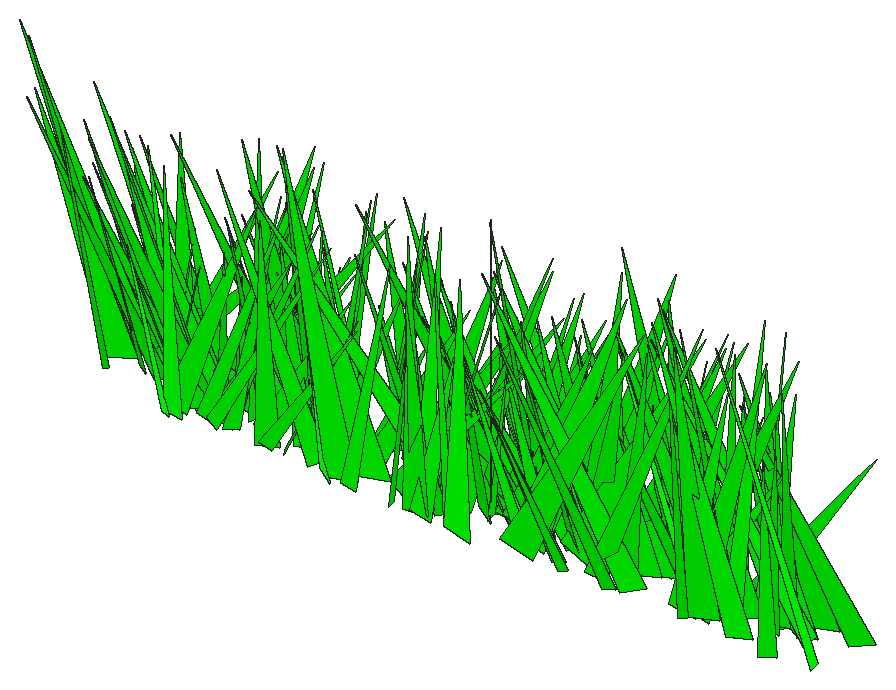
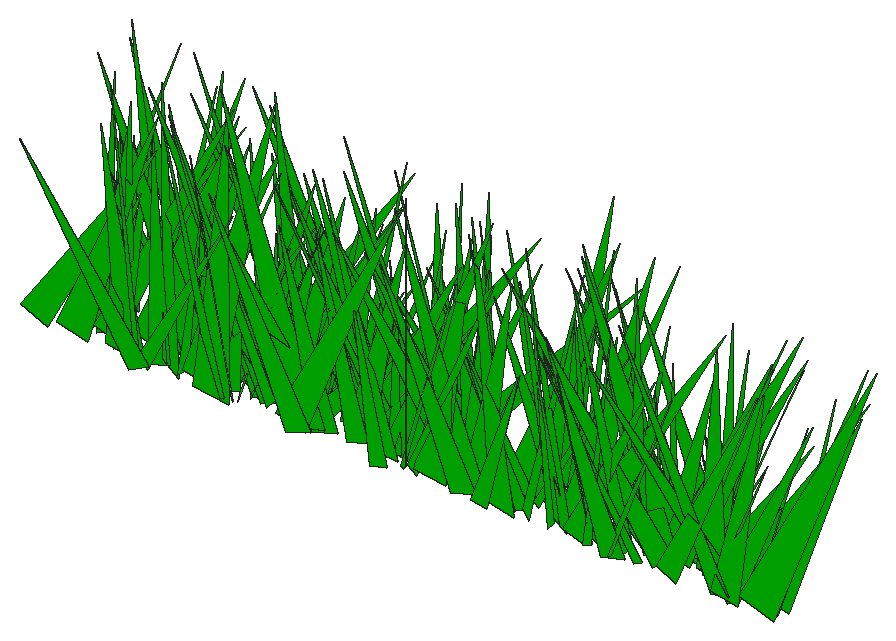
# SketchUp Ruby script. Lengths in inches.
U = 1.inch
M = Sketchup.active_model
def pt(a) = Geom::Point3d.new(a.map { |v| v * U })
def face(e, loops, mat)
  f = e.add_face(loops[0].map { |a| pt(a) })
  loops[1..].each { |l| e.add_face(l.map { |a| pt(a) }).erase! }
  f.material = f.back_material = mat if mat
  f
end
# faces: each face lists its corners as indices into pts; further lists are holes
def faces(e, pts, list, mat = nil) = list.each { |f| face(e, (f[0].is_a?(Array) ? f : [f]).map { |l| l.map { |i| pts[i] } }, mat) }
# xy, xz, yz: faces in a plane at the given z, y or x. An outline is a flat list of corners, or four numbers for a rectangle; further outlines are holes
def ring(l) = l.size == 4 ? [[l[0], l[1]], [l[2], l[1]], [l[2], l[3]], [l[0], l[3]]] : l.each_slice(2).to_a
def flat(e, list, mat, &to3) = list.each { |f| face(e, (f[0].is_a?(Array) ? f : [f]).map { |l| ring(l).map { |u, v| to3.(u, v) } }, mat) }
def xy(e, z, list, mat = nil) = flat(e, list, mat) { |x, y| [x, y, z] }
def xz(e, y, list, mat = nil) = flat(e, list, mat) { |x, z| [x, y, z] }
def yz(e, x, list, mat = nil) = flat(e, list, mat) { |y, z| [x, y, z] }
def lines(e, pts, list) = list.each { |a, b| e.add_line(pt(pts[a]), pt(pts[b])) }
# prism: a flat outline (further loops are holes) pulled along v
def prism(e, loops, v, mat = nil)
  f = face(e, loops, mat); d = Geom::Vector3d.new(v.map { |x| x * U })
  f.pushpull(f.normal.samedirection?(d) ? d.length : -d.length)
end
def box(e, o, s, mat = nil) = prism(e, [[o, [o[0] + s[0], o[1], o[2]], [o[0] + s[0], o[1] + s[1], o[2]], [o[0], o[1] + s[1], o[2]]]], [0, 0, s[2]], mat)
def at(x, y, z, deg = 0) = Geom::Transformation.translation(pt([x, y, z])) * Geom::Transformation.rotation(ORIGIN, Z_AXIS, deg.degrees)
def axes(o, x, y, z) = Geom::Transformation.new([*x, 0, *y, 0, *z, 0, *pt(o).to_a, 1])
def part(name) = M.definitions.add(name)
# library, detail: a bought-in or finely detailed component or shape, given as its bounding box
def library(name, o, s) = part(name).tap { |d| box(d.entities, o, s) }
def detail(e, o, s) = box(e.add_group.entities, o, s)
def put(e, d, t, mat = nil) = e.add_instance(d, t).tap { |i| i.material = mat if mat }
def group(e, t, mat = nil) = e.add_group.tap { |g| g.transformation = t; g.material = mat if mat }.entities
root = M.entities
M.materials.add("[0065_Lime]").color = [0, 255, 0]
c1 = part("fur_instance\#9")
p = [[0.8125,0,1.79],[0.67,-0.02,1.48],[0,-0.11,0],[0,0.11,0]]
faces(c1.entities,p,[[0,1,2,3]])
put(root,c1,axes([8.35,30.09,1.48],[-0.97184,-1.14595,3.29784],[8.52533,0.08708,2.67617],[-3.20375,0.57933,6.12105]),"[0065_Lime]")
put(root,c1,axes([8.03,29.625,1.48],[-7.32027,-0.64299,1.47519],[4.91342,-0.98176,1.79282],[0.29309,0.39896,6.7893]),"[0065_Lime]")
put(root,c1,axes([8.07,29.26,1.48],[-0.99814,1.05656,0.62338],[-7.15463,-0.09708,-2.06636],[-2.43606,-0.1478,5.81341]),"[0065_Lime]")
put(root,c1,axes([8.03,28.19,1.48],[-6.15676,-0.26004,1.50467],[2.26605,-0.86217,1.14185],[1.30829,0.26959,5.10315]),"[0065_Lime]")
put(root,c1,axes([10.48,28.9,1.48],[-6.27578,-0.65891,0.1631],[4.53982,-0.84028,1.82705],[-1.191,0.26908,6.10485]),"[0065_Lime]")
put(root,c1,axes([9.92,29.98,1.48],[-4.83605,-0.60584,1.73783],[4.78748,-0.56307,2.23707],[-0.48321,0.48463,4.77167]),"[0065_Lime]")
put(root,c1,axes([9.3,29.0625,1.48],[-5.32084,-0.29493,0.50758],[1.94317,-0.7422,-0.97326],[1.0093,-0.12587,4.54965]),"[0065_Lime]")
put(root,c1,axes([11.53,29.21,1.48],[-2.23326,-0.7401,0.77563],[4.95786,-0.2313,2.04934],[-2.01734,0.25086,4.17786]),"[0065_Lime]")
put(root,c1,axes([9.94,30.27,1.48],[1.48633,-0.93311,0.42277],[6.47605,0.21995,1.20288],[-1.55812,0.02405,5.40287]),"[0065_Lime]")
put(root,c1,axes([10.84,29.81,1.48],[-4.63654,0.19619,0.01665],[-1.34515,-0.63022,1.00372],[0.37476,0.16523,3.80867]),"[0065_Lime]")
put(root,c1,axes([12.09,28.28,1.48],[-7.31753,-0.35366,0.04909],[2.26762,-0.93721,-2.60519],[1.09369,-0.42308,5.72998]),"[0065_Lime]")
put(root,c1,axes([12.22,28.89,1.48],[-4.77681,-0.10309,0.28654],[0.81372,-0.59945,1.74818],[-0.01527,0.30602,3.52098]),"[0065_Lime]")
put(root,c1,axes([13.86,28.35,1.48],[-3.58464,1.16781,0.62225],[-8.02183,-0.44983,-2.28713],[-2.30306,-0.25086,6.99782]),"[0065_Lime]")
put(root,c1,axes([13.09,30.21,1.48],[-4.46996,-0.70372,1.31461],[5.21048,-0.55011,1.85446],[-0.73726,0.37878,5.13569]),"[0065_Lime]")
put(root,c1,axes([13.71,27.94,1.48],[-3.83914,-0.9369,0.49014],[6.48063,-0.49562,1.84029],[-1.67926,0.22925,5.98153]),"[0065_Lime]")
put(root,c1,axes([11.9,28.12,1.48],[-6.67185,0.3202,1.33269],[-2.00766,-0.9594,1.074],[1.96115,0.10716,5.6333]),"[0065_Lime]")
put(root,c1,axes([13.56,28.91,1.48],[-4.31946,0.82738,1.28636],[-6.02935,-0.53932,-1.77163],[-0.90401,-0.35625,5.66963]),"[0065_Lime]")
put(root,c1,axes([13.8,27.97,1.48],[-7.33696,-0.45983,1.01519],[3.49568,-0.98653,1.74213],[0.2157,0.347,6.29818]),"[0065_Lime]")
put(root,c1,axes([13.24,27.84,1.48],[-2.73427,0.90347,0.68486],[-6.37937,-0.35176,-1.30181],[-1.1627,-0.19463,5.53206]),"[0065_Lime]")
put(root,c1,axes([11.55,29.11,1.48],[2.14592,1.02268,0.75275],[-7.19215,0.31999,-1.00192],[-1.44846,-0.07376,6.09009]),"[0065_Lime]")
put(root,c1,axes([12.44,26.65,1.48],[-4.62827,0.19644,0.38265],[-1.25208,-0.63831,0.96033],[0.77968,0.14103,3.81362]),"[0065_Lime]")
put(root,c1,axes([11.1,28.67,1.48],[4.72564,0.21525,1.01076],[-1.0953,0.66336,-1.34548],[-1.64038,0.17715,3.81021]),"[0065_Lime]")
put(root,c1,axes([11.51,28.17,1.48],[4.07647,0.10586,0.77597],[-0.4582,0.56832,-1.00527],[-1.12588,0.15198,3.21866]),"[0065_Lime]")
put(root,c1,axes([12.72,26.81,1.48],[-6.19282,0.53477,1.31474],[-3.46206,-0.89428,1.39905],[2.26049,0.09541,5.74456]),"[0065_Lime]")
put(root,c1,axes([13.95,28.97,1.48],[1.44044,0.80035,1.96536],[-5.80563,0.29535,-1.21496],[-2.13868,-0.2627,4.62182]),"[0065_Lime]")
put(root,c1,axes([10.24,30.18,1.48],[5.66866,0.67536,0.71281],[-4.86771,0.76473,1.33372],[0.41577,-0.25463,5.89625]),"[0065_Lime]")
put(root,c1,axes([9.47,30,1.48],[5.43307,-0.59886,0.16116],[3.76874,0.65253,-2.81213],[1.99968,0.39726,4.86207]),"[0065_Lime]")
put(root,c1,axes([12.39,27.36,1.48],[3.44675,0.87455,0.94011],[-6.28399,0.45041,1.20327],[0.76337,-0.24099,5.66052]),"[0065_Lime]")
put(root,c1,axes([18.15,29.45,1.48],[-4.90993,-0.95425,0.12481],[6.5341,-0.65623,1.94955],[-1.85645,0.2141,6.53168]),"[0065_Lime]")
put(root,c1,axes([16.02,30.52,1.48],[-5.37657,-0.32663,0.09773],[2.19306,-0.72512,-1.38198],[0.77991,-0.21277,4.55978]),"[0065_Lime]")
put(root,c1,axes([14.16,28.37,1.48],[-4.55313,-0.58157,0.58505],[3.37137,-0.59481,-2.45291],[2.50612,-0.25644,4.36271]),"[0065_Lime]")
put(root,c1,axes([15.73,28.78,1.48],[6.82093,0.89005,0.74167],[-5.21382,0.88151,-3.7221],[-3.71052,0.3975,6.59349]),"[0065_Lime]")
put(root,c1,axes([15.48,27.5,1.48],[-4.21522,-0.04002,1.81893],[1.21862,-0.60101,1.42536],[1.89645,0.29724,3.127]),"[0065_Lime]")
put(root,c1,axes([13.24,28.53,1.48],[2.38102,-0.7524,0.33874],[5.15504,0.30222,-1.48046],[1.50641,0.155,4.53086]),"[0065_Lime]")
put(root,c1,axes([16.4375,28.5,1.48],[-6.08492,-0.64352,0.02362],[4.08332,-0.76542,-2.77695],[2.07369,-0.3811,5.53742]),"[0065_Lime]")
put(root,c1,axes([14.15,28.06,1.48],[2.05348,0.47895,0.93099],[-3.46149,0.21325,1.37543],[0.97245,-0.25229,2.92999]),"[0065_Lime]")
put(root,c1,axes([14.45,28.41,1.48],[-1.7297,0.78278,1.62237],[-5.40952,-0.32752,1.47931],[2.39753,-0.17423,4.5082]),"[0065_Lime]")
put(root,c1,axes([13.8125,28.89,1.48],[-2.12175,1.24777,1.08071],[-8.35474,-0.34463,2.48067],[3.28848,-0.07051,6.99969]),"[0065_Lime]")
put(root,c1,axes([13.96,27.4,1.48],[6.93903,-0.34959,1.35721],[2.87332,0.94403,-1.57158],[-0.84716,0.33839,5.7865]),"[0065_Lime]")
put(root,c1,axes([18.26,30.02,1.48],[-3.06513,-0.7045,0.61286],[4.978,-0.39475,1.26721],[-0.96112,0.20222,4.60887]),"[0065_Lime]")
put(root,c1,axes([15.41,27.34,1.48],[6.18285,0.7193,0.29128],[-4.82277,0.84146,-1.89736],[-1.75296,0.22202,6.24744]),"[0065_Lime]")
put(root,c1,axes([14.22,29.12,1.48],[1.43022,-1.18718,1.37587],[8.39868,0.13828,-1.77822],[1.92406,0.27886,6.73932]),"[0065_Lime]")
put(root,c1,axes([15.625,29.73,1.48],[7.6016,-0.16949,2.30745],[2.19241,1.04292,-2.21185],[-2.16687,0.46063,5.85686]),"[0065_Lime]")
put(root,c1,axes([17.32,30.27,1.48],[-5.76029,-0.40293,1.31263],[2.52516,-0.83445,-1.25126],[2.10948,-0.10138,5.08217]),"[0065_Lime]")
put(root,c1,axes([18.84,28.96,1.48],[-0.27338,-1.28528,0.61899],[8.99873,-0.01647,1.48349],[-1.80699,0.11242,7.29409]),"[0065_Lime]")
put(root,c1,axes([14.67,30.15,1.48],[5.23159,0.37079,0.12512],[-2.54466,0.69356,1.52598],[0.71503,-0.24467,4.51521]),"[0065_Lime]")
put(root,c1,axes([15,27.53,1.48],[7.1417,-0.28239,0.71473],[2.13405,0.99175,-0.97858],[-0.50648,0.19687,5.95489]),"[0065_Lime]")
put(root,c1,axes([17.51,27.16,1.48],[4.30859,-0.79145,1.16125],[5.47964,0.63653,1.0851],[-1.93272,0.04031,5.66524]),"[0065_Lime]")
put(root,c1,axes([20.11,27.35,1.48],[-7.23972,0.53248,2.02561],[-4.50893,-0.91517,-2.60122],[0.48002,-0.56553,6.11665]),"[0065_Lime]")
put(root,c1,axes([14.48,27.2,1.48],[6.67903,0.45508,0.10268],[-3.19482,0.9176,1.22384],[0.54532,-0.19784,5.91246]),"[0065_Lime]")
put(root,c1,axes([15.73,30.5,1.48],[1.529,-0.82776,0.08876],[5.69209,0.20344,-1.3002],[1.52098,0.07076,4.77662]),"[0065_Lime]")
put(root,c1,axes([18.83,28.04,1.48],[1.6355,0.7903,1.11266],[-5.53641,0.27186,-1.08601],[-1.68842,-0.12591,4.63887]),"[0065_Lime]")
put(root,c1,axes([13.81,29.5,1.48],[6.8052,-0.67836,0.68488],[4.63338,0.82476,-3.0874],[1.59572,0.49818,6.04392]),"[0065_Lime]")
put(root,c1,axes([17.36,29.91,1.48],[4.84983,0.15697,0.90715],[-0.78141,0.6787,-1.17119],[-1.3715,0.16838,3.87509]),"[0065_Lime]")
put(root,c1,axes([19.34,28.12,1.48],[-7.66578,-0.29747,2.32532],[2.66286,-1.11263,1.03878],[2.35858,0.28935,6.38489]),"[0065_Lime]")
put(root,c1,axes([21.11,28.9,1.48],[-6.1749,0.05928,0.23242],[-0.48996,-0.82484,-1.56297],[0.13987,-0.27227,4.78569]),"[0065_Lime]")
put(root,c1,axes([16.56,28.07,1.48],[3.45418,-0.54832,1.17075],[4.04515,0.38179,-1.90486],[0.96688,0.36157,3.78685]),"[0065_Lime]")
put(root,c1,axes([19.08,27.91,1.48],[-6.78528,0.34938,1.61231],[-1.06984,-0.86894,3.3307],[2.99443,0.48124,4.84343]),"[0065_Lime]")
put(root,c1,axes([20.9,29.87,1.48],[-7.92592,-0.06719,1.85351],[-0.5441,-1.05114,-2.81629],[2.26385,-0.48788,5.81242]),"[0065_Lime]")
put(root,c1,axes([19.46,29.98,1.48],[6.43506,-0.03039,2.05543],[0.66949,0.9544,-0.91394],[-2.4462,0.18126,5.15695]),"[0065_Lime]")
put(root,c1,axes([20.99,26.67,1.48],[-6.70839,0.34586,0.4284],[-1.75794,-0.79456,3.28141],[1.80143,0.51258,4.79752]),"[0065_Lime]")
put(root,c1,axes([22.72,27.76,1.48],[-4.34875,1.15919,0.44308],[-8.18068,-0.59086,-1.32588],[-1.19429,-0.17366,7.4687]),"[0065_Lime]")
put(root,c1,axes([17.46,27.11,1.48],[4.23747,-0.40977,0.14146],[2.81196,0.56045,-1.33044],[0.79197,0.20258,3.96701]),"[0065_Lime]")
put(root,c1,axes([21,28.5,1.48],[1.04393,0.83536,0.87042],[-5.82869,0.17936,-1.14276],[-1.58529,-0.10936,4.7748]),"[0065_Lime]")
put(root,c1,axes([19.41,29.57,1.48],[6.35941,0.75357,0.38742],[-4.90467,0.85359,-2.36755],[-2.22055,0.27276,6.33889]),"[0065_Lime]")
put(root,c1,axes([18.35,27.3,1.48],[5.32079,0.14556,0.0736],[-0.87563,0.66298,-2.05209],[-0.56077,0.34587,3.90262]),"[0065_Lime]")
put(root,c1,axes([18.78,29.875,1.48],[7.72117,-0.32797,1.20663],[1.89657,1.07786,1.78742],[-2.01275,-0.24249,6.31302]),"[0065_Lime]")
put(root,c1,axes([21.75,26.85,1.48],[4.51467,-0.94343,3.9011],[7.3073,0.81392,1.00059],[-3.83172,0.44062,6.50459]),"[0065_Lime]")
put(root,c1,axes([26.82,28.17,1.48],[-8.16704,0.64447,0.3537],[-4.03896,-0.9418,-4.2023],[-2.21613,-0.65861,6.35534]),"[0065_Lime]")
put(root,c1,axes([19.88,28.625,1.48],[3.8979,-0.61041,0.82337],[4.44674,0.51701,-1.08455],[0.34905,0.23006,4.62191]),"[0065_Lime]")
put(root,c1,axes([23,30.38,1.48],[1.58458,-0.51685,1.34756],[3.60867,0.2934,0.96318],[-1.80303,0.13299,3.11205]),"[0065_Lime]")
put(root,c1,axes([23.87,29.17,1.48],[0.41493,0.66008,0.0266],[-4.4172,0.05639,-1.30323],[-1.5987,0.0155,3.60771]),"[0065_Lime]")
put(root,c1,axes([23.875,29.48,1.48],[1.16109,0.99883,0.8784],[-6.94054,0.19583,-1.3918],[-1.87666,-0.10628,5.69082]),"[0065_Lime]")
put(root,c1,axes([21.27,29.64,1.48],[2.84389,-0.41734,0.81053],[3.11351,0.35563,-1.09206],[0.34638,0.22984,3.16147]),"[0065_Lime]")
put(root,c1,axes([21.69,29.86,1.48],[7.7133,-0.13283,1.39072],[0.39371,1.0641,1.96077],[-1.91355,-0.31647,6.00923]),"[0065_Lime]")
put(root,c1,axes([21.93,30.1875,1.48],[7.13168,-0.75006,0.34518],[5.02392,0.97164,2.07066],[-1.85268,-0.25246,6.94374]),"[0065_Lime]")
put(root,c1,axes([22.35,26.53,1.48],[-5.44394,0.48822,2.5686],[-3.06686,-0.88422,1.331],[3.55494,-0.01518,5.08174]),"[0065_Lime]")
put(root,c1,axes([26.88,27.14,1.48],[-5.98853,-0.51302,1.3565],[4.01365,-0.7621,2.06567],[-0.03149,0.42689,5.31792]),"[0065_Lime]")
put(root,c1,axes([21.9375,28.56,1.48],[3.90133,0.69755,0.5187],[-4.87641,0.50419,1.54685],[1.12707,-0.23314,4.89719]),"[0065_Lime]")
put(root,c1,axes([25.01,28.52,1.48],[-3.23815,-0.79996,0.21531],[5.56486,-0.45305,-1.02969],[1.22964,-0.0563,5.22695]),"[0065_Lime]")
put(root,c1,axes([24.66,26.53,1.48],[7.02796,0.39612,1.58276],[-1.98769,0.97988,-2.37806],[-2.78968,0.29977,5.6818]),"[0065_Lime]")
put(root,c1,axes([27.01,29.85,1.48],[-6.60531,0.15787,1.161],[-1.61392,-0.85715,-2.16983],[0.83346,-0.40867,4.99944]),"[0065_Lime]")
put(root,c1,axes([26.07,29.85,1.48],[1.18692,-1.08328,0.55749],[7.60368,0.18139,1.09983],[-1.44424,0.06472,6.24861]),"[0065_Lime]")
put(root,c1,axes([25.26,27.91,1.48],[-6.5462,0.65941,1.87174],[-4.12926,-0.97021,1.89831],[3.20408,0.09688,6.27058]),"[0065_Lime]")
put(root,c1,axes([25.91,26.59,1.48],[4.01921,0.9489,1.83256],[-6.75036,0.62346,-1.02197],[-2.26056,-0.17461,6.30998]),"[0065_Lime]")
put(root,c1,axes([28.21,29.2,1.48],[-3.46825,1.05096,1.76825],[-7.68471,-0.40727,-1.86163],[-1.26869,-0.40615,6.44239]),"[0065_Lime]")
put(root,c1,axes([30.18,28.54,1.48],[-4.6697,-1.07849,0.66095],[7.18469,-0.55869,3.03766],[-2.81926,0.36259,6.64651]),"[0065_Lime]")
put(root,c1,axes([25.98,26.94,1.48],[3.5297,-0.79968,0.80723],[5.49481,0.51519,1.2052],[-1.78299,0.00463,5.31219]),"[0065_Lime]")
put(root,c1,axes([27.48,29.93,1.48],[-6.09029,-0.01921,1.06648],[-0.11809,-0.85944,-0.96496],[1.31293,-0.16642,4.86031]),"[0065_Lime]")
put(root,c1,axes([23.96,29.75,1.48],[3.71289,-0.97413,0.65811],[6.93333,0.49999,-1.08124],[0.80148,0.18743,6.30474]),"[0065_Lime]")
put(root,c1,axes([24.06,30.09,1.48],[1.83716,-0.86839,0.27806],[5.89685,0.23035,-1.67165],[1.88034,0.12605,4.9707]),"[0065_Lime]")
put(root,c1,axes([23.45,29.54,1.48],[3.29252,-0.79681,1.04707],[5.44113,0.34888,-2.42421],[2.05078,0.35363,4.75086]),"[0065_Lime]")
put(root,c1,axes([26.25,26.51,1.48],[-1.66468,0.72538,0.1718],[-4.9552,-0.23299,1.1958],[1.46261,0.03626,4.24681]),"[0065_Lime]")
put(root,c1,axes([29.8,29.02,1.48],[-3.29145,0.64193,0.14188],[-4.26007,-0.41971,-1.75662],[-1.65883,-0.19584,4.22971]),"[0065_Lime]")
put(root,c1,axes([28.62,29.0625,1.48],[-5.3949,-0.00903,0.53924],[-0.14926,-0.72454,-1.39459],[0.6491,-0.24166,4.16112]),"[0065_Lime]")
put(root,c1,axes([28.7,28.65,1.48],[-0.88588,0.6097,0.88633],[-4.29235,-0.07185,-1.18235],[-1.26076,-0.18378,3.4026]),"[0065_Lime]")
put(root,c1,axes([27.21,27.13,1.48],[7.51815,-0.32487,2.17258],[1.08619,1.05238,2.78615],[-3.36142,-0.38654,5.75947]),"[0065_Lime]")
put(root,c1,axes([27.69,29.42,1.48],[7.52708,0.25201,2.73217],[-0.95885,1.13736,-1.76759],[-3.68501,0.21882,6.04072]),"[0065_Lime]")
put(root,c1,axes([23.86,27.79,1.48],[4.4593,0.63315,0.06722],[-4.04079,0.55452,2.34257],[1.99534,-0.29204,4.59372]),"[0065_Lime]")
put(root,c1,axes([30.33,28.65,1.48],[-2.32091,0.94008,0.40617],[-6.42437,-0.29005,-1.79317],[-1.93237,-0.16478,5.47374]),"[0065_Lime]")
put(root,c1,axes([28.29,28.28,1.48],[-5.97201,-0.58669,0.58169],[3.66642,-0.8029,-2.23018],[2.12155,-0.26392,5.49159]),"[0065_Lime]")
put(root,c1,axes([29.87,28.51,1.48],[-0.79362,0.60258,0.57517],[-3.88619,-0.05316,-1.6816],[-1.94606,-0.13958,3.1235]),"[0065_Lime]")
put(root,c1,axes([24.68,29.24,1.48],[1.54533,0.99838,0.39241],[-6.45379,0.16701,2.57712],[3.01042,-0.15445,5.32343]),"[0065_Lime]")
put(root,c1,axes([28.43,26.22,1.48],[-5.58116,0.87314,0.02744],[-5.84817,-0.74025,2.27292],[2.10011,0.25906,6.40232]),"[0065_Lime]")
put(root,c1,axes([25.98,27.68,1.48],[8.00409,-0.10995,0.92791],[0.46827,1.10104,1.69907],[-1.30164,-0.27999,6.31716]),"[0065_Lime]")
put(root,c1,axes([28.45,29.24,1.48],[-3.57968,-0.50529,1.0955],[3.41811,-0.5372,-0.91293],[1.74959,0.01568,4.02496]),"[0065_Lime]")
put(root,c1,axes([26.59,28.38,1.48],[0.90385,1.17557,0.84456],[-8.125,0.08235,1.91214],[2.24779,-0.17503,6.57211]),"[0065_Lime]")
put(root,c1,axes([30.84,28.03,1.48],[-5.15692,0.04234,0.29568],[-0.39074,-0.6972,-1.16348],[0.26506,-0.20401,4.03757]),"[0065_Lime]")
put(root,c1,axes([30.49,29.11,1.48],[0.86474,0.98177,0.93734],[-6.77393,0.16222,-1.55881],[-2.06337,-0.12112,5.5103]),"[0065_Lime]")
put(root,c1,axes([26.03,29.06,1.48],[8.96809,-0.42259,0.13632],[2.91516,1.23635,1.54049],[-0.75791,-0.24502,7.53821]),"[0065_Lime]")
put(root,c1,axes([28.32,30.48,1.48],[-1.36852,-0.64412,0.4739],[4.33533,-0.20853,-1.2139],[1.59891,0.0141,3.69704]),"[0065_Lime]")
put(root,c1,axes([28.65,28.27,1.48],[5.24529,-0.2608,0.78629],[1.34649,0.70123,1.85056],[-1.60189,-0.26454,4.13017]),"[0065_Lime]")
put(root,c1,axes([30.46,29.26,1.48],[-4.28313,-0.19375,0.30307],[1.17534,-0.57216,-1.26653],[0.81153,-0.19393,3.43391]),"[0065_Lime]")
put(root,c1,axes([30.47,28.8,1.48],[-2.85652,-0.37613,1.34459],[3.14162,-0.35766,1.06337],[0.16663,0.29521,3.00146]),"[0065_Lime]")
put(root,c1,axes([31.39,27.06,1.48],[-4.86675,0.30155,0.99676],[-2.42419,-0.65643,-1.17677],[0.47997,-0.25773,4.16335]),"[0065_Lime]")
put(root,c1,axes([33.02,28.42,1.48],[-3.59085,0.54376,0.3759],[-3.45096,-0.40262,-2.29539],[-1.81079,-0.31098,3.62909]),"[0065_Lime]")
put(root,c1,axes([31.72,28.06,1.48],[-8.49554,-0.26923,2.22169],[2.74372,-1.16116,2.22661],[1.89821,0.4734,6.72492]),"[0065_Lime]")
put(root,c1,axes([28.48,29.625,1.48],[6.9788,-0.55309,0.1623],[3.84463,0.96795,1.1516],[-0.86678,-0.15978,6.41473]),"[0065_Lime]")
put(root,c1,axes([33.54,29.84,1.48],[-3.21088,1.0221,1.04202],[-7.16466,-0.38338,-2.00618],[-1.7936,-0.29832,6.14841]),"[0065_Lime]")
put(root,c1,axes([31.96,27.89,1.48],[-0.63053,0.63997,1.14986],[-4.66123,-0.04041,-0.93758],[-1.00684,-0.21372,3.6205]),"[0065_Lime]")
put(root,c1,axes([31.54,28.36,1.48],[-4.4899,-0.72538,0.71531],[5.00449,-0.64231,-1.04216],[1.54158,-0.02753,5.46658]),"[0065_Lime]")
put(root,c1,axes([33.26,27.03,1.48],[-3.00403,-0.53635,0.2002],[3.71196,-0.3982,1.10485],[-0.92259,0.14429,3.79338]),"[0065_Lime]")
put(root,c1,axes([29.46,28.57,1.48],[2.53884,1.03367,0.99495],[-7.41012,0.32933,1.04561],[0.83646,-0.2199,6.243]),"[0065_Lime]")
put(root,c1,axes([28.65,29,1.48],[0.9695,1.00442,1.28863],[-6.8824,0.04843,2.16095],[2.49732,-0.25645,5.45512]),"[0065_Lime]")
put(root,c1,axes([30.27,29.46,1.48],[3.79968,-0.56715,1.94463],[4.65513,0.50927,-1.04108],[-0.57955,0.37225,4.38716]),"[0065_Lime]")
put(root,c1,axes([28.37,29.125,1.48],[8.0356,0.07166,0.08759],[-0.44455,1.0643,-2.19424],[-0.27213,0.37743,6.1709]),"[0065_Lime]")
put(root,c1,axes([35.14,28.34,1.48],[-3.29932,1.03517,0.64237],[-7.05774,-0.40215,-2.2684],[-2.25439,-0.25598,6.1615]),"[0065_Lime]")
put(root,c1,axes([33.29,28.13,1.48],[-5.81012,-0.40513,0.42956],[2.74028,-0.80926,-1.05178],[1.04022,-0.13097,5.16999]),"[0065_Lime]")
put(root,c1,axes([33.83,26.58,1.48],[-3.09662,-0.40046,0.3915],[2.8027,-0.39185,1.23648],[-0.70586,0.2009,3.19207]),"[0065_Lime]")
put(root,c1,axes([33.52,28.5625,1.48],[-0.50965,0.87579,1.37839],[-6.31074,-0.01666,-1.18905],[-1.37521,-0.24809,4.94565]),"[0065_Lime]")
put(root,c1,axes([29.91,28.38,1.48],[-1.07145,-1.06191,0.46591],[6.89783,-0.17031,-2.51199],[3.13975,0.01179,5.67766]),"[0065_Lime]")
put(root,c1,axes([31.89,29.63,1.48],[-1.96702,0.9073,0.25711],[-6.18075,-0.27756,1.53407],[1.89453,0.03652,5.27173]),"[0065_Lime]")
put(root,c1,axes([34.76,28.41,1.48],[-4.05618,0.46124,0.7017],[-3.37445,-0.52791,-1.27841],[-0.36265,-0.24672,4.04723]),"[0065_Lime]")
put(root,c1,axes([37.2,27.11,1.48],[-6.32788,0.84857,0.54383],[-5.83901,-0.81184,-2.50493],[-1.67958,-0.37467,6.6594]),"[0065_Lime]")
put(root,c1,axes([34.46,28.91,1.48],[-0.0511,-1.00185,0.69071],[7.03562,0.01683,1.16231],[-1.43302,0.11835,5.68187]),"[0065_Lime]")
put(root,c1,axes([36.34,26.53,1.48],[-5.54104,-0.59741,0.35608],[4.17789,-0.73588,1.64491],[-0.90098,0.26173,5.43763]),"[0065_Lime]")
put(root,c1,axes([31.43,28.11,1.48],[4.79891,0.57098,0.75557],[-4.16583,0.65031,1.03891],[0.14016,-0.22104,5.00822]),"[0065_Lime]")
put(root,c1,axes([31.13,27.52,1.48],[1.54474,1.17416,1.91783],[-8.40225,0.1174,2.06924],[2.18707,-0.37828,6.59501]),"[0065_Lime]")
put(root,c1,axes([35.18,28.73,1.48],[1.7303,0.76517,1.79278],[-5.43567,0.33098,-1.26243],[-2.22774,-0.21327,4.4728]),"[0065_Lime]")
put(root,c1,axes([36.31,28.98,1.48],[-6.55783,-0.0114,0.53816],[0.27265,-0.8848,1.57016],[0.60825,0.2737,5.09832]),"[0065_Lime]")
put(root,c1,axes([31.92,29.53,1.48],[0.97577,0.83667,0.67043],[-5.41692,0.07153,2.22495],[2.60558,-0.16461,4.37454]),"[0065_Lime]")
put(root,c1,axes([31.22,26.74,1.48],[4.08579,-1.10673,0.92983],[7.67302,0.49984,-2.37217],[2.11297,0.32493,6.81628]),"[0065_Lime]")
put(root,c1,axes([33.82,28.45,1.48],[-3.06919,-1.11445,2.57043],[8.1684,-0.52056,-1.10956],[2.48285,0.33496,6.82785]),"[0065_Lime]")
put(root,c1,axes([36.55,29.54,1.48],[-5.63737,0.0224,0.6358],[0.05291,-0.77167,1.22152],[0.79598,0.20996,4.42172]),"[0065_Lime]")
put(root,c1,axes([36.92,28.44,1.48],[-2.88863,0.88059,1.44504],[-6.47151,-0.35697,-1.2701],[-0.7399,-0.31567,5.46732]),"[0065_Lime]")
put(root,c1,axes([34.01,28.37,1.48],[-1.05162,-1.02749,0.61309],[7.13474,-0.16843,-1.36126],[1.76957,0.06846,5.85279]),"[0065_Lime]")
put(root,c1,axes([32.77,29.8,1.48],[2.78372,-1.24026,1.4499],[8.88529,0.33581,-1.6614],[1.46081,0.3209,7.34248]),"[0065_Lime]")
put(root,c1,axes([33.06,29.29,1.48],[5.80444,-0.6565,1.50705],[5.02208,0.77323,-1.51102],[-0.19748,0.36762,5.86946]),"[0065_Lime]")
put(root,c1,axes([32.75,30.32,1.48],[2.37286,-0.84663,0.94609],[5.89575,0.26596,-1.80838],[1.70137,0.25913,4.9471]),"[0065_Lime]")
put(root,c1,axes([35.7,28.08,1.48],[3.56538,0.63246,0.36579],[-4.09063,0.48517,-1.72888],[-1.93057,0.14,4.33882]),"[0065_Lime]")
put(root,c1,axes([37.7,28.88,1.48],[-1.40832,0.70734,0.69583],[-4.92812,-0.15568,-1.29655],[-1.33594,-0.1714,4.04929]),"[0065_Lime]")
put(root,c1,axes([39.03,28.61,1.48],[-4.98341,-0.54486,0.19994],[3.75985,-0.66212,1.54127],[-0.97942,0.23053,4.89938]),"[0065_Lime]")
put(root,c1,axes([38.68,29.44,1.48],[-0.06269,1.17525,3.4209],[-9.11231,0.1278,-1.58169],[-2.14577,-0.57705,6.61691]),"[0065_Lime]")
put(root,c1,axes([35.98,28.1,1.48],[-3.56311,-0.84921,1.64903],[5.87315,-0.56421,-1.33971],[2.47769,0.11619,5.54709]),"[0065_Lime]")
put(root,c1,axes([33.25,28.04,1.48],[5.1097,0.97049,1.13992],[-6.86302,0.63001,2.38133],[1.60099,-0.39673,6.56997]),"[0065_Lime]")
put(root,c1,axes([37.07,29.33,1.48],[-4.30904,-0.65592,0.05533],[4.18503,-0.54851,-2.24382],[2.06861,-0.25661,4.65478]),"[0065_Lime]")
put(root,c1,axes([40.01,27.7,1.48],[-7.40669,0.29099,0.07127],[-1.96135,-0.99874,1.78042],[0.67031,0.29305,5.99705]),"[0065_Lime]")
put(root,c1,axes([37.61,30.09,1.48],[3.71068,-1.1972,0.03232],[8.35644,0.51259,1.46022],[-1.66143,-0.0957,7.41659]),"[0065_Lime]")
put(root,c1,axes([35.16,29.16,1.48],[8.1331,-0.12603,0.88871],[1.14061,1.1147,-1.60934],[-0.83497,0.29512,6.45818]),"[0065_Lime]")
put(root,c1,axes([36.65,29.89,1.48],[6.73322,0.02798,1.3893],[-0.6062,0.94629,1.30529],[-1.60915,-0.23941,5.32154]),"[0065_Lime]")
put(root,c1,axes([35.59,28.93,1.48],[2.41069,1.04733,0.80737],[-7.35955,0.29864,1.55809],[1.54093,-0.21217,6.17843]),"[0065_Lime]")
put(root,c1,axes([35.22,27.02,1.48],[8.17614,-0.55794,1.00951],[4.13276,1.13334,-1.15698],[-0.47552,0.2567,7.30224]),"[0065_Lime]")
put(root,c1,axes([41.12,28.08,1.48],[-0.64554,-1.02675,2.50148],[7.36609,0.0826,2.39377],[-2.93075,0.43376,5.46547]),"[0065_Lime]")
put(root,c1,axes([35.05,28.95,1.48],[5.01779,-0.97142,1.30934],[6.92457,0.60906,-2.41624],[1.55977,0.42113,6.51471]),"[0065_Lime]")
put(root,c1,axes([37.27,30.04,1.48],[6.52048,0.45338,1.6692],[-3.61985,0.91556,1.02283],[-1.23212,-0.29051,5.8286]),"[0065_Lime]")
put(root,c1,axes([40.88,28.08,1.48],[-4.21331,0.80953,1.37384],[-6.00082,-0.55918,-1.13552],[-0.18014,-0.30686,5.69347]),"[0065_Lime]")
put(root,c1,axes([39.76,29.31,1.48],[-5.04222,0.33775,0.63619],[-2.06358,-0.69167,1.48341],[1.45973,0.18888,4.29461]),"[0065_Lime]")
put(root,c1,axes([41.59,29.65,1.48],[-5.57488,-0.37627,0.74333],[2.81497,-0.70904,1.94184],[-0.28493,0.35695,4.64076]),"[0065_Lime]")
put(root,c1,axes([39.39,28.84,1.48],[3.01167,-0.49326,0.77969],[3.27752,0.44367,1.02887],[-1.58074,-0.01987,3.61876]),"[0065_Lime]")
put(root,c1,axes([39.27,28.3,1.48],[-3.21518,0.49538,0.69625],[-3.32392,-0.46665,0.96983],[1.45351,0.02865,3.75795]),"[0065_Lime]")
put(root,c1,axes([40.27,26.5625,1.48],[-6.4199,-0.30403,2.60357],[3.14411,-0.91805,1.53728],[2.2452,0.41627,5.29185]),"[0065_Lime]")
put(root,c1,axes([38.99,28.55,1.48],[4.84721,-0.38775,0.63962],[2.48771,0.67602,1.25874],[-1.4297,-0.13832,4.3588]),"[0065_Lime]")
put(root,c1,axes([42.39,28.26,1.48],[0.44439,1.25359,1.14142],[-8.43893,0.12794,-2.53474],[-3.21591,-0.16251,6.80917]),"[0065_Lime]")
put(root,c1,axes([38.86,28,1.48],[4.23779,0.05227,0.3638],[-0.17349,0.55466,-1.33315],[-0.55524,0.22561,3.1932]),"[0065_Lime]")
put(root,c1,axes([41.02,27.04,1.48],[3.96957,-1.06055,1.11704],[7.30749,0.58888,1.55312],[-2.33469,0.03995,6.76044]),"[0065_Lime]")
put(root,c1,axes([43.22,26.69,1.48],[-6.42671,0.80154,1.37001],[-5.9421,-0.88032,-1.18434],[0.25654,-0.31076,6.88862]),"[0065_Lime]")
put(root,c1,axes([42.51,27.39,1.48],[-7.29798,-0.47084,1.90808],[3.78864,-1.03223,1.05252],[1.54148,0.30788,6.44671]),"[0065_Lime]")
put(root,c1,axes([44.32,28.75,1.48],[-6.87345,0.74939,1.35539],[-5.55455,-0.87634,-2.40131],[-0.6042,-0.46872,6.65662]),"[0065_Lime]")
put(root,c1,axes([39.91,27.02,1.48],[3.17939,-0.7716,2.60398],[6.35317,0.40115,-1.14934],[-0.19419,0.49095,5.03161]),"[0065_Lime]")
put(root,c1,axes([40.32,29.43,1.48],[8.46009,-0.56683,0.95663],[2.98695,1.0726,3.81883],[-2.95525,-0.53859,6.59838]),"[0065_Lime]")
put(root,c1,axes([40.93,29.45,1.48],[-3.76703,-0.83999,0.62712],[5.59011,-0.53467,-1.78055],[2.25375,-0.07782,5.46461]),"[0065_Lime]")
put(root,c1,axes([40,27.97,1.48],[5.91399,0.44329,0.24092],[-2.97663,0.80748,-1.43979],[-1.08594,0.20078,5.25858]),"[0065_Lime]")
put(root,c1,axes([45.72,28.31,1.48],[-8.25478,0.37618,0.18345],[-2.5645,-1.07282,-2.6349],[-0.80061,-0.4422,6.54861]),"[0065_Lime]")
put(root,c1,axes([39.5,28.13,1.48],[2.74751,0.68135,0.04295],[-4.61479,0.36478,1.41533],[1.48919,-0.12667,4.30667]),"[0065_Lime]")
put(root,c1,axes([38.97,28.9,1.48],[4.85614,-1.04181,0.63597],[7.36254,0.64957,-1.54018],[1.1716,0.23613,7.04273]),"[0065_Lime]")
put(root,c1,axes([42.93,26.76,1.48],[-4.57486,-0.0524,1.09004],[0.90485,-0.60374,1.54011],[1.05647,0.29018,3.40115]),"[0065_Lime]")
put(root,c1,axes([40.42,27.18,1.48],[4.22901,0.96871,2.53626],[-7.56008,0.52083,1.67474],[0.3042,-0.5233,6.36184]),"[0065_Lime]")
put(root,c1,axes([42.09,29.5,1.48],[7.65278,0.41867,1.93873],[-2.33684,1.10765,-1.91216],[-3.01619,0.2041,6.4005]),"[0065_Lime]")
put(root,c1,axes([43.13,29.22,1.48],[-5.92553,-0.69913,0.17402],[4.439,-0.76268,-2.66674],[2.25738,-0.33543,5.70076]),"[0065_Lime]")
put(root,c1,axes([42.15,27.47,1.48],[8.24481,-0.3945,3.00401],[3.62795,1.20785,-1.27293],[-2.89116,0.39066,6.96929]),"[0065_Lime]")
put(root,c1,axes([43.78,28.48,1.48],[3.17988,0.98669,1.13148],[-6.85961,0.48116,-1.30492],[-2.04626,-0.07966,6.13275]),"[0065_Lime]")
put(root,c1,axes([42.72,29.19,1.48],[-2.54301,0.87205,1.29108],[-6.14818,-0.39964,1.03278],[1.79827,-0.13313,5.35677]),"[0065_Lime]")
put(root,c1,axes([43.29,29.48,1.48],[5.08175,-0.55148,1.19398],[3.56507,0.73942,1.40466],[-2.20168,-0.07558,5.03033]),"[0065_Lime]")
put(root,c1,axes([44.4,28.67,1.48],[1.11343,0.97741,0.49985],[-6.83268,0.17053,-1.10385],[-1.4404,-0.05341,5.62261]),"[0065_Lime]")
put(root,c1,axes([45.52,29.51,1.48],[-0.43885,-1.11561,0.10846],[7.68905,-0.05502,1.62036],[-1.98217,0.03356,6.26153]),"[0065_Lime]")
put(root,c1,axes([45.49,28.43,1.48],[-0.86211,0.72672,0.17827],[-4.9934,-0.10853,-1.15246],[-1.36406,-0.06201,4.10613]),"[0065_Lime]")
put(root,c1,axes([43.68,28.11,1.48],[-2.85185,-0.72383,0.68385],[4.91439,-0.41774,-1.25636],[1.75794,-0.00646,4.6216]),"[0065_Lime]")
put(root,c1,axes([44.42,28.65,1.48],[-6.02938,-0.81162,0.86868],[5.07243,-0.82789,-2.62487],[2.96176,-0.23437,6.26387]),"[0065_Lime]")
put(root,c1,axes([47.64,29.4,1.48],[-0.1678,-1.0216,0.35164],[6.50299,0.00634,2.6708],[-3.27947,0.06485,5.27805]),"[0065_Lime]")
put(root,c1,axes([41.42,30.18,1.48],[4.45281,-0.63738,0.16254],[4.26281,0.57334,-1.92879],[1.56311,0.25212,4.79705]),"[0065_Lime]")
put(root,c1,axes([47.21,26.74,1.48],[-8.8791,0.09354,1.09731],[-0.89082,-1.24138,-1.22345],[1.21219,-0.22713,7.13856]),"[0065_Lime]")
put(root,c1,axes([45.15,26.15,1.48],[3.09908,0.7406,0.3318],[-4.93736,0.42926,-1.59383],[-1.88868,0.09307,4.711]),"[0065_Lime]")
